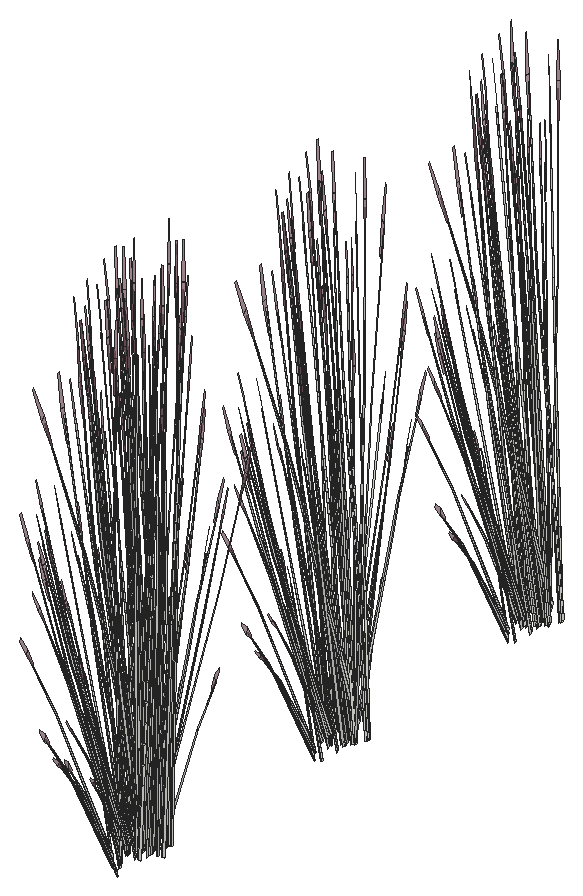
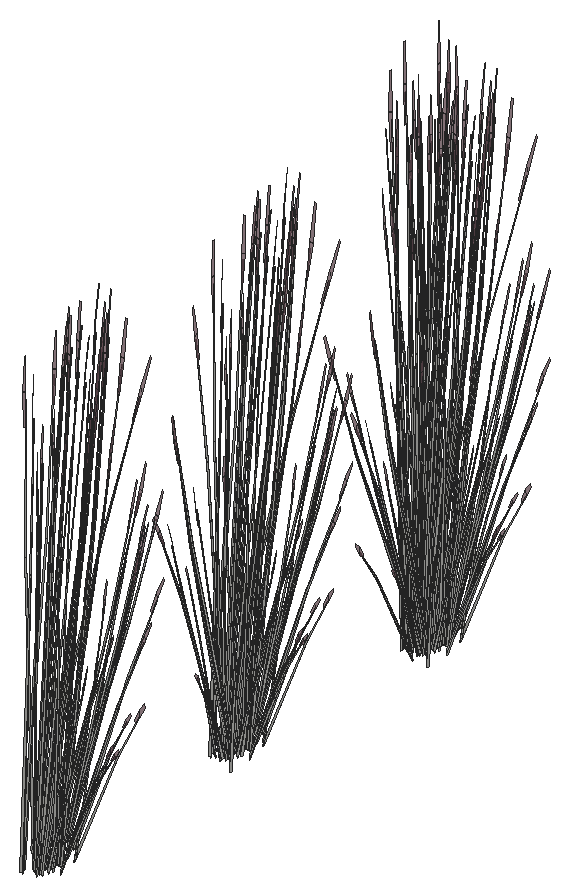
# SketchUp Ruby script. Lengths in inches.
U = 1.inch
M = Sketchup.active_model
def pt(a) = Geom::Point3d.new(a.map { |v| v * U })
def face(e, loops, mat)
  f = e.add_face(loops[0].map { |a| pt(a) })
  loops[1..].each { |l| e.add_face(l.map { |a| pt(a) }).erase! }
  f.material = f.back_material = mat if mat
  f
end
# faces: each face lists its corners as indices into pts; further lists are holes
def faces(e, pts, list, mat = nil) = list.each { |f| face(e, (f[0].is_a?(Array) ? f : [f]).map { |l| l.map { |i| pts[i] } }, mat) }
# xy, xz, yz: faces in a plane at the given z, y or x. An outline is a flat list of corners, or four numbers for a rectangle; further outlines are holes
def ring(l) = l.size == 4 ? [[l[0], l[1]], [l[2], l[1]], [l[2], l[3]], [l[0], l[3]]] : l.each_slice(2).to_a
def flat(e, list, mat, &to3) = list.each { |f| face(e, (f[0].is_a?(Array) ? f : [f]).map { |l| ring(l).map { |u, v| to3.(u, v) } }, mat) }
def xy(e, z, list, mat = nil) = flat(e, list, mat) { |x, y| [x, y, z] }
def xz(e, y, list, mat = nil) = flat(e, list, mat) { |x, z| [x, y, z] }
def yz(e, x, list, mat = nil) = flat(e, list, mat) { |y, z| [x, y, z] }
def lines(e, pts, list) = list.each { |a, b| e.add_line(pt(pts[a]), pt(pts[b])) }
# prism: a flat outline (further loops are holes) pulled along v
def prism(e, loops, v, mat = nil)
  f = face(e, loops, mat); d = Geom::Vector3d.new(v.map { |x| x * U })
  f.pushpull(f.normal.samedirection?(d) ? d.length : -d.length)
end
def box(e, o, s, mat = nil) = prism(e, [[o, [o[0] + s[0], o[1], o[2]], [o[0] + s[0], o[1] + s[1], o[2]], [o[0], o[1] + s[1], o[2]]]], [0, 0, s[2]], mat)
def at(x, y, z, deg = 0) = Geom::Transformation.translation(pt([x, y, z])) * Geom::Transformation.rotation(ORIGIN, Z_AXIS, deg.degrees)
def axes(o, x, y, z) = Geom::Transformation.new([*x, 0, *y, 0, *z, 0, *pt(o).to_a, 1])
def part(name) = M.definitions.add(name)
# library, detail: a bought-in or finely detailed component or shape, given as its bounding box
def library(name, o, s) = part(name).tap { |d| box(d.entities, o, s) }
def detail(e, o, s) = box(e.add_group.entities, o, s)
def put(e, d, t, mat = nil) = e.add_instance(d, t).tap { |i| i.material = mat if mat }
def group(e, t, mat = nil) = e.add_group.tap { |g| g.transformation = t; g.material = mat if mat }.entities
root = M.entities
M.materials.add("LightPink_Translucent").color = [144, 107, 117]
M.materials["LightPink_Translucent"].alpha = 0.75
c1 = part("blade")
p = [[2.15,0.21,22],[0,0.17,0],[0.09,0.45,0],[2.18,0.31,22],[2.29,0.31,22],[0.38,0.45,0],
  [2.48,0.24,33],[2.49,0.24,33],[2.48,0.22,33]]
faces(c1.entities,p,[[0,1,2,3],[4,5,2,3],[6,3,4,7],[8,0,3,6]])
c2 = part("seeds")
p = [[0.3,-0.1,1.38],[-0.01,-0.03,1.59],[-0.01,-0.03,0.03],[0.14,-0.07,-0.07],[0.29,-0.03,3],[0.15,0.01,3.11]]
faces(c2.entities,p,[[0,1,2,3],[1,0,4,5]],"LightPink_Translucent")
c3 = part("blade with seeds")
put(c3.entities,c1,at(0,0,0))
put(c3.entities,c2,axes([2.4,0.25,30.99],[1.5799,-0.05474,1.17369],[-0.12525,1.92788,0.29478],[-0.07173,-0.02425,1.56792]))
put(root,c3,axes([431.11,19.21,2.28],[-0.17959,-0.44867,-0.61099],[0.36969,-0.25004,0.07373],[-0.042,-0.21679,0.8643]))
put(root,c3,axes([429.9375,18.61,0.23],[-0.02279,0.18051,1.22981],[-0.33311,0.15111,-0.26449],[-0.07787,-0.23331,0.52581]))
put(root,c3,axes([430.8,18.21,-0.72],[-0.06312,0.01988,1.51654],[-0.34903,-0.22379,-0.23168],[0.00586,-0.18666,0.25832]))
put(root,c3,axes([431.14,18.83,1.89],[0.11344,-0.42434,-0.30456],[0.33096,0.12377,0.39319],[-0.03035,-0.17085,0.75234]))
put(root,c3,axes([430.97,19.12,2.03],[-0.3699,-0.13833,-0.43945],[0.12679,-0.47426,-0.34039],[-0.03392,-0.19095,0.84085]))
put(root,c3,axes([431.2,17.93,0.38],[0.04827,0.32177,0.9878],[-0.26778,-0.17821,0.72577],[0.02882,-0.16476,0.21757]))
put(root,c3,axes([429.82,18.32,0.38],[0.19628,0.19205,0.9878],[-0.28586,0.11545,0.72577],[-0.06116,-0.1476,0.21757]))
put(root,c3,axes([430.3,19.34,2.28],[-0.32086,-0.26671,-0.61099],[0.22803,-0.46737,0.07373],[-0.11625,-0.15925,0.8643]))
put(root,c3,axes([430.1875,18.98,1.89],[-0.05812,-0.44446,-0.30456],[0.33222,-0.11736,0.39319],[-0.08923,-0.12737,0.75234]))
put(root,c3,axes([429.67,18.9,-0.72],[-0.03645,0.07269,1.51654],[-0.36835,0.15672,-0.23168],[-0.08898,-0.14257,0.25832]))
put(root,c3,axes([430.28,20.9,-0.2],[-0.15453,-0.56584,-0.60058],[0.44514,-0.20379,-0.15763],[-0.01708,-0.19161,1.32568]))
put(root,c3,axes([430.15,19.35,2.03],[-0.37131,0.13117,-0.43945],[-0.06495,-0.49674,-0.34039],[-0.09973,-0.14235,0.84085]))
put(root,c3,axes([430.21,19.27,0.04],[-0.23526,-0.55293,0],[0.3936,-0.30836,-0.44382],[0.08964,-0.07023,1.40792]))
put(root,c3,axes([430.73,18.6,-0.17],[-0.26003,0.31656,-0.03348],[-0.23826,-0.3467,-0.15179],[-0.01677,-0.09824,0.50065]))
put(root,c3,axes([431.06,22.35,0.86],[0.32517,0.22251,1.30084],[-0.31856,0.47936,0.51441],[-0.14269,-0.28411,1.09053]))
put(root,c3,axes([429.36,20.82,-0.26],[0,-0.5518,-0.427],[0.42099,0,0],[0,-0.12568,1.35453]))
put(root,c3,axes([430.51,21.04,-0.1],[0.18257,-0.49721,-0.38476],[0.37935,0.23929,0.18517],[0,-0.11462,1.23533]))
put(root,c3,axes([429.42,19.77,1.89],[-0.2141,-0.34548,-0.30456],[0.24447,-0.32704,0.39319],[-0.12421,-0.04976,0.75234]))
put(root,c3,axes([429.55,20.83,-0.26],[0.26266,-0.34428,-0.26641],[0.26266,0.34428,0.26641],[0,-0.11089,1.19518]))
put(root,c3,axes([429.4375,19.18,-0.17],[-0.10855,0.45057,-0.03348],[-0.33409,-0.1386,-0.15179],[-0.05073,-0.0737,0.50065]))
put(root,c3,axes([430.47,21.45,0.29],[-0.42377,-0.26329,-0.25022],[0.20405,-0.55571,-0.43002],[-0.01332,-0.13644,1.37348]))
put(root,c3,axes([429.26,21.23,0.04],[-0.47052,0,0],[0,-0.61671,-0.44382],[0,-0.14046,1.40792]))
put(root,c3,axes([429.34,20.13,0.23],[0.07347,0.15363,1.22981],[-0.16929,0.41759,-0.26449],[-0.17383,-0.09981,0.52581]))
put(root,c3,axes([429.64,20,2.28],[-0.37615,-0.01329,-0.61099],[0.02526,-0.55946,0.07373],[-0.15935,-0.05904,0.8643]))
put(root,c3,axes([429.625,21.07,0],[-0.35001,0.46392,0.2645],[-0.35022,-0.45904,-0.31383],[-0.01222,-0.13174,1.41801]))
put(root,c3,axes([430.74,21.29,0.09],[0.42398,0.26744,0.20696],[-0.20405,0.55571,0.43002],[0,-0.1281,1.38067]))
put(root,c3,axes([430.57,22.04,0.1],[0.09973,-0.65385,-0.20149],[0.47288,0.11397,0.44093],[-0.08263,-0.0903,1.34539]))
put(root,c3,axes([429.52,20.11,2.03],[-0.27323,0.36552,-0.43945],[-0.23929,-0.38612,-0.34039],[-0.13882,-0.05561,0.84085]))
put(root,c3,axes([428.9,20.59,0.38],[0.24023,-0.03948,0.9878],[-0.15239,0.3479,0.72577],[-0.11872,-0.05219,0.21757]))
put(root,c3,axes([430.6,20.92,0.34],[-0.40861,0.03406,0.38476],[-0.03695,-0.56543,-0.18517],[0.07315,-0.05731,1.23533]))
put(root,c3,axes([429.55,21.33,0.13],[0,0.5518,0.427],[-0.42099,0,0],[0,-0.12568,1.35453]))
put(root,c3,axes([430.54,21.77,-0.1],[-0.22605,-0.46315,-0.38476],[0.34239,-0.32614,0.18517],[-0.07315,-0.05731,1.23533]))
put(root,c3,axes([430.59,21.12,0.03],[0.1636,0.61702,0.39349],[-0.46745,0.21456,0.15441],[0.00571,-0.11338,1.36617]))
put(root,c3,axes([430.5,21.61,0.34],[-0.18257,0.49721,0.38476],[-0.37935,-0.23929,-0.18517],[0,-0.11462,1.23533]))
put(root,c3,axes([431.17,21.17,-0.1],[0,-0.63847,0],[0.47052,0,0],[0,0,1.54332]))
put(root,c3,axes([430.34,21.95,-0.23],[-0.39143,-0.09047,-0.53624],[0.0826,-0.55804,-0.14074],[-0.11681,-0.06762,1.18365]))
put(root,c3,axes([430.95,20.77,0.03],[-0.312,0.50076,0.39349],[-0.37066,-0.44204,0.15441],[0.07522,-0.04998,1.36617]))
put(root,c3,axes([431.29,21.67,-0.02],[-0.35001,-0.47494,-0.05273],[0.35022,-0.47523,0],[-0.01222,-0.01659,1.50991]))
put(root,c3,axes([430.41,19.95,0.13],[-0.1087,0.54839,0.15172],[-0.39778,-0.15519,0.30174],[0.06871,-0.00267,1.3795]))
put(root,c3,axes([430.625,21.72,0.03],[0.4756,0.11626,0.39349],[-0.09679,0.6566,0.15441],[-0.0695,-0.0634,1.36617]))
put(root,c3,axes([429.08,21.16,-0.72],[0.00954,0.08696,1.51654],[-0.19238,0.45414,-0.23168],[-0.13665,-0.02289,0.25832]))
put(root,c3,axes([429.92,22.8,-0.26],[-0.08839,-0.48081,-0.26641],[0.35106,-0.13653,0.26641],[-0.07077,-0.05545,1.19518]))
put(root,c3,axes([430.37,22.77,0.13],[0.40434,-0.14646,0.15172],[0.09984,0.54504,0.30174],[-0.03606,-0.07941,1.3795]))
put(root,c3,axes([429.82,23.01,-0.26],[-0.35217,-0.2759,-0.427],[0.2105,-0.49473,0],[-0.08021,-0.06284,1.35453]))
put(root,c3,axes([429.04,20.97,1.89],[-0.31272,-0.15393,-0.30456],[0.09121,-0.44909,0.39319],[-0.1259,0.04118,0.75234]))
put(root,c3,axes([430.78,22.03,0.29],[-0.37992,0.36634,-0.25022],[-0.25264,-0.51764,-0.43002],[-0.09374,-0.05257,1.37348]))
put(root,c3,axes([431.61,19.98,0.13],[-0.40434,0.14646,0.15172],[-0.09984,-0.54504,0.30174],[0.03606,0.07941,1.3795]))
put(root,c3,axes([430.98,22.65,-0.1],[-0.12277,-0.47573,0],[0.35059,-0.1666,0],[0,0,1.32759]))
put(root,c3,axes([430.74,22.19,0.25],[-0.07259,0.49245,0.12452],[-0.35466,-0.08548,-0.35559],[-0.06454,-0.05057,1.09]))
put(root,c3,axes([431.57,22.8,0.13],[0.1087,-0.54839,0.15172],[0.39778,0.15519,0.30174],[-0.06871,0.00267,1.3795]))
put(root,c3,axes([429.99,20.89,0.875],[0.10696,-0.07982,1.52275],[0.03688,0.55733,0.11917],[-0.23167,0.07395,0.54424]))
put(root,c3,axes([432.2,21.4,0.13],[-0.29564,-0.40194,0.15172],[0.29793,-0.38985,0.30174],[-0.03265,0.08208,1.3795]))
put(root,c3,axes([430.89,22.86,-0.11],[-0.37935,-0.24773,0],[0.18257,-0.51475,0],[0,0,1.39928]))
put(root,c3,axes([431.21,22.2,0.12],[-0.36743,-0.44413,-0.21665],[0.30918,-0.49872,0.47412],[-0.09894,0.05195,1.44665]))
put(root,c3,axes([430.24,23.05,0.13],[0.35217,0.2759,0.427],[-0.2105,0.49473,0],[-0.08021,-0.06284,1.35453]))
put(root,c3,axes([431.41,21.43,-0.03],[0,0.63816,-0.04848],[-0.47052,0,0],[0,0.02005,1.54256]))
put(root,c3,axes([429.25,21.19,2.03],[-0.10194,0.50193,-0.43945],[-0.34951,-0.17204,-0.34039],[-0.14072,0.04602,0.84085]))
put(root,c3,axes([430.04,23.34,0.04],[-0.23526,0.55293,0],[-0.3936,-0.30836,-0.44382],[-0.08964,-0.07023,1.40792]))
put(root,c3,axes([431.38,21.83,0.34],[0.40861,-0.03406,0.38476],[0.03695,0.56543,-0.18517],[-0.07315,0.05731,1.23533]))
put(root,c3,axes([431.02,22.11,-0.1],[-0.40861,0.03406,-0.38476],[-0.03695,-0.56543,0.18517],[-0.07315,0.05731,1.23533]))
put(root,c3,axes([431.47,23.42,-0.11],[-0.23233,-0.55486,-0.04422],[0.3936,-0.30836,0.44382],[-0.09699,0.05283,1.40722]))
put(root,c3,axes([431.39,22.08,0.25],[0.278,0.33153,0.12452],[-0.23189,0.37404,-0.35559],[-0.06454,0.05057,1.09]))
put(root,c3,axes([431.6875,23.1,0.13],[0.35217,-0.2759,0.427],[0.2105,0.49473,0],[-0.08021,0.06284,1.35453]))
put(root,c3,axes([431.1875,22.66,-0.03],[0.1636,0.63392,-0.05171],[-0.46745,0.22213,0],[0.00571,0.02214,1.48069]))
put(root,c3,axes([431.37,23.35,-0.26],[-0.35106,-0.13653,-0.26641],[0.08839,-0.48081,0.26641],[-0.07077,0.05545,1.19518]))
put(root,c3,axes([428.83,22.37,0.23],[0.13077,0.0453,1.22981],[0.08428,0.46268,-0.26449],[-0.17763,0.08661,0.52581]))
put(root,c3,axes([432.54,21.83,-0.11],[-0.47029,-0.00441,-0.0428],[0,-0.61671,0.42951],[-0.01478,0.14039,1.36183]))
put(root,c3,axes([428.5625,23.34,0.38],[0.15682,-0.25009,0.9878],[0.06188,0.39591,0.72577],[-0.11333,0.07089,0.21757]))
put(root,c3,axes([431.31,21.95,0.29],[0.04385,0.62963,-0.25022],[-0.45669,0.03807,-0.43002],[-0.08042,0.08387,1.37348]))
put(root,c3,axes([431.47,21.71,-0.1],[-0.18257,0.49721,-0.38476],[-0.37935,-0.23929,0.18517],[0,0.11462,1.23533]))
put(root,c3,axes([429.15,22.26,1.89],[-0.32754,0.07886,-0.30456],[-0.08649,-0.45081,0.39319],[-0.09386,0.12109,0.75234]))
put(root,c3,axes([431.03,22.43,-0.23],[-0.25345,0.41475,-0.53624],[-0.31485,-0.37608,-0.14074],[-0.10156,0.10346,1.18365]))
put(root,c3,axes([431.48,23.13,0],[0.47108,0.17935,0.2645],[-0.11785,0.64108,-0.31383],[-0.07797,0.08023,1.41801]))
put(root,c3,axes([431.45,23.57,-0.26],[-0.35217,0.2759,-0.427],[-0.2105,-0.49473,0],[-0.08021,0.06284,1.35453]))
put(root,c3,axes([429.42,22.3125,2.03],[0.09666,0.50384,-0.43945],[-0.36608,0.08814,-0.34039],[-0.10491,0.13533,0.84085]))
put(root,c3,axes([431.77,23.48,0.04],[0.23526,0.55293,0],[-0.3936,0.30836,-0.44382],[-0.08964,0.07023,1.40792]))
put(root,c3,axes([431.57,21.29,0.44],[-0.01028,-0.51954,1.21494],[0.46521,0.13467,0.51441],[-0.11003,0.28429,1.14681]))
put(root,c3,axes([428.97,23.6,-0.72],[0.05047,0.05513,1.51654],[0.08558,0.51079,-0.23168],[-0.11187,0.10892,0.25832]))
put(root,c3,axes([429.73,23.3,1.89],[-0.2546,0.29052,-0.30456],[-0.24101,-0.33173,0.39319],[-0.03667,0.16855,0.75234]))
put(root,c3,axes([429.89,24.43,0.38],[-0.00974,-0.3281,0.9878],[0.24334,0.23402,0.72577],[-0.04786,0.15639,0.21757]))
put(root,c3,axes([430.53,23.65,-0.72],[0.0609,-0.03003,1.51654],[0.36632,0.16527,-0.23168],[0.01071,0.18627,0.25832]))
put(root,c3,axes([429.98,23.17,2.3],[0.26937,0.37076,-0.48779],[-0.28456,0.3247,-0.37783],[-0.04099,0.18838,0.93334]))
put(root,c3,axes([429.69,23.72,0.43],[0.34184,-0.09771,0.05596],[0.07859,0.39367,-0.74222],[-0.02167,0.19928,0.6653]))
put(root,c3,axes([430.61,23.82,1.89],[-0.11344,0.42434,-0.30456],[-0.33096,-0.12377,0.39319],[0.03035,0.17085,0.75234]))
put(root,c3,axes([429.9,23,2.59],[-0.00979,0.51041,-0.6782],[-0.4123,-0.03428,0.08184],[-0.04351,0.21623,0.95938]))
put(root,c3,axes([430.65,23.4375,2.28],[0.17959,0.44867,-0.61099],[-0.36969,0.25004,0.07373],[0.042,0.21679,0.8643]))
put(root,c3,axes([429.61,24.14,0.23],[0.11874,-0.08705,1.22981],[0.29317,0.26247,-0.26449],[-0.08726,0.22711,0.52581]))
put(root,c3,axes([429.76,23.72,0.89],[0.00827,-0.28486,1.32737],[0.37184,0.15046,0.18343],[-0.03222,0.30359,0.62678]))
put(root,c3,axes([432.74,42.25,2.28],[-0.17959,-0.44867,-0.61099],[0.36969,-0.25004,0.07373],[-0.042,-0.21679,0.8643]))
put(root,c3,axes([431.57,41.65,0.23],[-0.02279,0.18051,1.22981],[-0.33311,0.15111,-0.26449],[-0.07787,-0.23331,0.52581]))
put(root,c3,axes([432.6,42.16,2.03],[-0.3699,-0.13833,-0.43945],[0.12679,-0.47426,-0.34039],[-0.03392,-0.19095,0.84085]))
put(root,c3,axes([431.45,41.36,0.38],[0.19628,0.19205,0.9878],[-0.28586,0.11545,0.72577],[-0.06116,-0.1476,0.21757]))
put(root,c3,axes([431.93,42.38,2.28],[-0.32086,-0.26671,-0.61099],[0.22803,-0.46737,0.07373],[-0.11625,-0.15925,0.8643]))
put(root,c3,axes([431.82,42.03,1.89],[-0.05812,-0.44446,-0.30456],[0.33222,-0.11736,0.39319],[-0.08923,-0.12737,0.75234]))
put(root,c3,axes([431.3,41.94,-0.72],[-0.03645,0.07269,1.51654],[-0.36835,0.15672,-0.23168],[-0.08898,-0.14257,0.25832]))
put(root,c3,axes([431.9,43.9375,-0.2],[-0.15453,-0.56584,-0.60058],[0.44514,-0.20379,-0.15763],[-0.01708,-0.19161,1.32568]))
put(root,c3,axes([431.78,42.39,2.03],[-0.37131,0.13117,-0.43945],[-0.06495,-0.49674,-0.34039],[-0.09973,-0.14235,0.84085]))
put(root,c3,axes([432.36,41.64,-0.17],[-0.26003,0.31656,-0.03348],[-0.23826,-0.3467,-0.15179],[-0.01677,-0.09824,0.50065]))
put(root,c3,axes([432.69,45.4,0.86],[0.32517,0.22251,1.30084],[-0.31856,0.47936,0.51441],[-0.14269,-0.28411,1.09053]))
put(root,c3,axes([430.99,43.86,-0.26],[0,-0.5518,-0.427],[0.42099,0,0],[0,-0.12568,1.35453]))
put(root,c3,axes([431.05,42.81,1.89],[-0.2141,-0.34548,-0.30456],[0.24447,-0.32704,0.39319],[-0.12421,-0.04976,0.75234]))
put(root,c3,axes([431.17,43.87,-0.26],[0.26266,-0.34428,-0.26641],[0.26266,0.34428,0.26641],[0,-0.11089,1.19518]))
put(root,c3,axes([431.07,42.22,-0.17],[-0.10855,0.45057,-0.03348],[-0.33409,-0.1386,-0.15179],[-0.05073,-0.0737,0.50065]))
put(root,c3,axes([432.09,44.5,0.29],[-0.42377,-0.26329,-0.25022],[0.20405,-0.55571,-0.43002],[-0.01332,-0.13644,1.37348]))
put(root,c3,axes([430.89,44.28,0.04],[-0.47052,0,0],[0,-0.61671,-0.44382],[0,-0.14046,1.40792]))
put(root,c3,axes([430.97,43.17,0.23],[0.07347,0.15363,1.22981],[-0.16929,0.41759,-0.26449],[-0.17383,-0.09981,0.52581]))
put(root,c3,axes([431.27,43.04,2.28],[-0.37615,-0.01329,-0.61099],[0.02526,-0.55946,0.07373],[-0.15935,-0.05904,0.8643]))
put(root,c3,axes([431.25,44.11,0],[-0.35001,0.46392,0.2645],[-0.35022,-0.45904,-0.31383],[-0.01222,-0.13174,1.41801]))
put(root,c3,axes([432.2,45.08,0.1],[0.09973,-0.65385,-0.20149],[0.47288,0.11397,0.44093],[-0.08263,-0.0903,1.34539]))
put(root,c3,axes([431.15,43.15,2.03],[-0.27323,0.36552,-0.43945],[-0.23929,-0.38612,-0.34039],[-0.13882,-0.05561,0.84085]))
put(root,c3,axes([430.53,43.64,0.38],[0.24023,-0.03948,0.9878],[-0.15239,0.3479,0.72577],[-0.11872,-0.05219,0.21757]))
put(root,c3,axes([431.17,44.37,0.13],[0,0.5518,0.427],[-0.42099,0,0],[0,-0.12568,1.35453]))
put(root,c3,axes([432.17,44.82,-0.1],[-0.22605,-0.46315,-0.38476],[0.34239,-0.32614,0.18517],[-0.07315,-0.05731,1.23533]))
put(root,c3,axes([432.13,44.65,0.34],[-0.18257,0.49721,0.38476],[-0.37935,-0.23929,-0.18517],[0,-0.11462,1.23533]))
put(root,c3,axes([431.97,44.99,-0.23],[-0.39143,-0.09047,-0.53624],[0.0826,-0.55804,-0.14074],[-0.11681,-0.06762,1.18365]))
put(root,c3,axes([432.26,44.77,0.03],[0.4756,0.11626,0.39349],[-0.09679,0.6566,0.15441],[-0.0695,-0.0634,1.36617]))
put(root,c3,axes([430.71,44.2,-0.72],[0.00954,0.08696,1.51654],[-0.19238,0.45414,-0.23168],[-0.13665,-0.02289,0.25832]))
put(root,c3,axes([431.55,45.84,-0.26],[-0.08839,-0.48081,-0.26641],[0.35106,-0.13653,0.26641],[-0.07077,-0.05545,1.19518]))
put(root,c3,axes([431.45,46.05,-0.26],[-0.35217,-0.2759,-0.427],[0.2105,-0.49473,0],[-0.08021,-0.06284,1.35453]))
put(root,c3,axes([430.67,44.01,1.89],[-0.31272,-0.15393,-0.30456],[0.09121,-0.44909,0.39319],[-0.1259,0.04118,0.75234]))
put(root,c3,axes([432.41,45.08,0.29],[-0.37992,0.36634,-0.25022],[-0.25264,-0.51764,-0.43002],[-0.09374,-0.05257,1.37348]))
put(root,c3,axes([432.375,45.24,0.25],[-0.07259,0.49245,0.12452],[-0.35466,-0.08548,-0.35559],[-0.06454,-0.05057,1.09]))
put(root,c3,axes([431.62,43.93,0.875],[0.10696,-0.07982,1.52275],[0.03688,0.55733,0.11917],[-0.23167,0.07395,0.54424]))
put(root,c3,axes([432.84,45.24,0.12],[-0.36743,-0.44413,-0.21665],[0.30918,-0.49872,0.47412],[-0.09894,0.05195,1.44665]))
put(root,c3,axes([431.87,46.09,0.13],[0.35217,0.2759,0.427],[-0.2105,0.49473,0],[-0.08021,-0.06284,1.35453]))
put(root,c3,axes([430.88,44.24,2.03],[-0.10194,0.50193,-0.43945],[-0.34951,-0.17204,-0.34039],[-0.14072,0.04602,0.84085]))
put(root,c3,axes([431.67,46.38,0.04],[-0.23526,0.55293,0],[-0.3936,-0.30836,-0.44382],[-0.08964,-0.07023,1.40792]))
put(root,c3,axes([432.65,45.15,-0.1],[-0.40861,0.03406,-0.38476],[-0.03695,-0.56543,0.18517],[-0.07315,0.05731,1.23533]))
put(root,c3,axes([433.1,46.46,-0.11],[-0.23233,-0.55486,-0.04422],[0.3936,-0.30836,0.44382],[-0.09699,0.05283,1.40722]))
put(root,c3,axes([433,46.39,-0.26],[-0.35106,-0.13653,-0.26641],[0.08839,-0.48081,0.26641],[-0.07077,0.05545,1.19518]))
put(root,c3,axes([430.46,45.41,0.23],[0.13077,0.0453,1.22981],[0.08428,0.46268,-0.26449],[-0.17763,0.08661,0.52581]))
put(root,c3,axes([430.19,46.38,0.38],[0.15682,-0.25009,0.9878],[0.06188,0.39591,0.72577],[-0.11333,0.07089,0.21757]))
put(root,c3,axes([432.9375,44.99,0.29],[0.04385,0.62963,-0.25022],[-0.45669,0.03807,-0.43002],[-0.08042,0.08387,1.37348]))
put(root,c3,axes([430.78,45.3,1.89],[-0.32754,0.07886,-0.30456],[-0.08649,-0.45081,0.39319],[-0.09386,0.12109,0.75234]))
put(root,c3,axes([432.66,45.48,-0.23],[-0.25345,0.41475,-0.53624],[-0.31485,-0.37608,-0.14074],[-0.10156,0.10346,1.18365]))
put(root,c3,axes([433.08,46.61,-0.26],[-0.35217,0.2759,-0.427],[-0.2105,-0.49473,0],[-0.08021,0.06284,1.35453]))
put(root,c3,axes([431.05,45.35,2.03],[0.09666,0.50384,-0.43945],[-0.36608,0.08814,-0.34039],[-0.10491,0.13533,0.84085]))
put(root,c3,axes([433.2,44.33,0.44],[-0.01028,-0.51954,1.21494],[0.46521,0.13467,0.51441],[-0.11003,0.28429,1.14681]))
put(root,c3,axes([430.6,46.64,-0.72],[0.05047,0.05513,1.51654],[0.08558,0.51079,-0.23168],[-0.11187,0.10892,0.25832]))
put(root,c3,axes([431.36,46.35,1.89],[-0.2546,0.29052,-0.30456],[-0.24101,-0.33173,0.39319],[-0.03667,0.16855,0.75234]))
put(root,c3,axes([431.52,47.47,0.38],[-0.00974,-0.3281,0.9878],[0.24334,0.23402,0.72577],[-0.04786,0.15639,0.21757]))
put(root,c3,axes([431.61,46.21,2.3],[0.26937,0.37076,-0.48779],[-0.28456,0.3247,-0.37783],[-0.04099,0.18838,0.93334]))
put(root,c3,axes([431.32,46.76,0.43],[0.34184,-0.09771,0.05596],[0.07859,0.39367,-0.74222],[-0.02167,0.19928,0.6653]))
put(root,c3,axes([431.53,46.04,2.59],[-0.00979,0.51041,-0.6782],[-0.4123,-0.03428,0.08184],[-0.04351,0.21623,0.95938]))
put(root,c3,axes([431.24,47.18,0.23],[0.11874,-0.08705,1.22981],[0.29317,0.26247,-0.26449],[-0.08726,0.22711,0.52581]))
put(root,c3,axes([431.39,46.76,0.89],[0.00827,-0.28486,1.32737],[0.37184,0.15046,0.18343],[-0.03222,0.30359,0.62678]))
put(root,c3,axes([432.74,66.25,2.28],[-0.17959,-0.44867,-0.61099],[0.36969,-0.25004,0.07373],[-0.042,-0.21679,0.8643]))
put(root,c3,axes([431.57,65.65,0.23],[-0.02279,0.18051,1.22981],[-0.33311,0.15111,-0.26449],[-0.07787,-0.23331,0.52581]))
put(root,c3,axes([432.6,66.16,2.03],[-0.3699,-0.13833,-0.43945],[0.12679,-0.47426,-0.34039],[-0.03392,-0.19095,0.84085]))
put(root,c3,axes([431.45,65.36,0.38],[0.19628,0.19205,0.9878],[-0.28586,0.11545,0.72577],[-0.06116,-0.1476,0.21757]))
put(root,c3,axes([431.93,66.38,2.28],[-0.32086,-0.26671,-0.61099],[0.22803,-0.46737,0.07373],[-0.11625,-0.15925,0.8643]))
put(root,c3,axes([431.82,66.03,1.89],[-0.05812,-0.44446,-0.30456],[0.33222,-0.11736,0.39319],[-0.08923,-0.12737,0.75234]))
put(root,c3,axes([431.3,65.94,-0.72],[-0.03645,0.07269,1.51654],[-0.36835,0.15672,-0.23168],[-0.08898,-0.14257,0.25832]))
put(root,c3,axes([431.9,67.9375,-0.2],[-0.15453,-0.56584,-0.60058],[0.44514,-0.20379,-0.15763],[-0.01708,-0.19161,1.32568]))
put(root,c3,axes([431.78,66.39,2.03],[-0.37131,0.13117,-0.43945],[-0.06495,-0.49674,-0.34039],[-0.09973,-0.14235,0.84085]))
put(root,c3,axes([432.36,65.64,-0.17],[-0.26003,0.31656,-0.03348],[-0.23826,-0.3467,-0.15179],[-0.01677,-0.09824,0.50065]))
put(root,c3,axes([432.69,69.4,0.86],[0.32517,0.22251,1.30084],[-0.31856,0.47936,0.51441],[-0.14269,-0.28411,1.09053]))
put(root,c3,axes([430.99,67.86,-0.26],[0,-0.5518,-0.427],[0.42099,0,0],[0,-0.12568,1.35453]))
put(root,c3,axes([431.05,66.81,1.89],[-0.2141,-0.34548,-0.30456],[0.24447,-0.32704,0.39319],[-0.12421,-0.04976,0.75234]))
put(root,c3,axes([431.17,67.87,-0.26],[0.26266,-0.34428,-0.26641],[0.26266,0.34428,0.26641],[0,-0.11089,1.19518]))
put(root,c3,axes([431.07,66.22,-0.17],[-0.10855,0.45057,-0.03348],[-0.33409,-0.1386,-0.15179],[-0.05073,-0.0737,0.50065]))
put(root,c3,axes([432.09,68.5,0.29],[-0.42377,-0.26329,-0.25022],[0.20405,-0.55571,-0.43002],[-0.01332,-0.13644,1.37348]))
put(root,c3,axes([430.89,68.28,0.04],[-0.47052,0,0],[0,-0.61671,-0.44382],[0,-0.14046,1.40792]))
put(root,c3,axes([430.97,67.17,0.23],[0.07347,0.15363,1.22981],[-0.16929,0.41759,-0.26449],[-0.17383,-0.09981,0.52581]))
put(root,c3,axes([431.27,67.04,2.28],[-0.37615,-0.01329,-0.61099],[0.02526,-0.55946,0.07373],[-0.15935,-0.05904,0.8643]))
put(root,c3,axes([431.25,68.11,0],[-0.35001,0.46392,0.2645],[-0.35022,-0.45904,-0.31383],[-0.01222,-0.13174,1.41801]))
put(root,c3,axes([432.2,69.08,0.1],[0.09973,-0.65385,-0.20149],[0.47288,0.11397,0.44093],[-0.08263,-0.0903,1.34539]))
put(root,c3,axes([431.15,67.15,2.03],[-0.27323,0.36552,-0.43945],[-0.23929,-0.38612,-0.34039],[-0.13882,-0.05561,0.84085]))
put(root,c3,axes([430.53,67.64,0.38],[0.24023,-0.03948,0.9878],[-0.15239,0.3479,0.72577],[-0.11872,-0.05219,0.21757]))
put(root,c3,axes([431.17,68.37,0.13],[0,0.5518,0.427],[-0.42099,0,0],[0,-0.12568,1.35453]))
put(root,c3,axes([432.17,68.82,-0.1],[-0.22605,-0.46315,-0.38476],[0.34239,-0.32614,0.18517],[-0.07315,-0.05731,1.23533]))
put(root,c3,axes([432.13,68.65,0.34],[-0.18257,0.49721,0.38476],[-0.37935,-0.23929,-0.18517],[0,-0.11462,1.23533]))
put(root,c3,axes([431.97,68.99,-0.23],[-0.39143,-0.09047,-0.53624],[0.0826,-0.55804,-0.14074],[-0.11681,-0.06762,1.18365]))
put(root,c3,axes([432.26,68.77,0.03],[0.4756,0.11626,0.39349],[-0.09679,0.6566,0.15441],[-0.0695,-0.0634,1.36617]))
put(root,c3,axes([430.71,68.2,-0.72],[0.00954,0.08696,1.51654],[-0.19238,0.45414,-0.23168],[-0.13665,-0.02289,0.25832]))
put(root,c3,axes([431.55,69.84,-0.26],[-0.08839,-0.48081,-0.26641],[0.35106,-0.13653,0.26641],[-0.07077,-0.05545,1.19518]))
put(root,c3,axes([431.45,70.05,-0.26],[-0.35217,-0.2759,-0.427],[0.2105,-0.49473,0],[-0.08021,-0.06284,1.35453]))
put(root,c3,axes([430.67,68.01,1.89],[-0.31272,-0.15393,-0.30456],[0.09121,-0.44909,0.39319],[-0.1259,0.04118,0.75234]))
put(root,c3,axes([432.41,69.08,0.29],[-0.37992,0.36634,-0.25022],[-0.25264,-0.51764,-0.43002],[-0.09374,-0.05257,1.37348]))
put(root,c3,axes([432.375,69.24,0.25],[-0.07259,0.49245,0.12452],[-0.35466,-0.08548,-0.35559],[-0.06454,-0.05057,1.09]))
put(root,c3,axes([431.62,67.93,0.875],[0.10696,-0.07982,1.52275],[0.03688,0.55733,0.11917],[-0.23167,0.07395,0.54424]))
put(root,c3,axes([432.84,69.24,0.12],[-0.36743,-0.44413,-0.21665],[0.30918,-0.49872,0.47412],[-0.09894,0.05195,1.44665]))
put(root,c3,axes([431.87,70.09,0.13],[0.35217,0.2759,0.427],[-0.2105,0.49473,0],[-0.08021,-0.06284,1.35453]))
put(root,c3,axes([430.88,68.24,2.03],[-0.10194,0.50193,-0.43945],[-0.34951,-0.17204,-0.34039],[-0.14072,0.04602,0.84085]))
put(root,c3,axes([431.67,70.38,0.04],[-0.23526,0.55293,0],[-0.3936,-0.30836,-0.44382],[-0.08964,-0.07023,1.40792]))
put(root,c3,axes([432.65,69.15,-0.1],[-0.40861,0.03406,-0.38476],[-0.03695,-0.56543,0.18517],[-0.07315,0.05731,1.23533]))
put(root,c3,axes([433.1,70.46,-0.11],[-0.23233,-0.55486,-0.04422],[0.3936,-0.30836,0.44382],[-0.09699,0.05283,1.40722]))
put(root,c3,axes([433,70.39,-0.26],[-0.35106,-0.13653,-0.26641],[0.08839,-0.48081,0.26641],[-0.07077,0.05545,1.19518]))
put(root,c3,axes([430.46,69.41,0.23],[0.13077,0.0453,1.22981],[0.08428,0.46268,-0.26449],[-0.17763,0.08661,0.52581]))
put(root,c3,axes([430.19,70.38,0.38],[0.15682,-0.25009,0.9878],[0.06188,0.39591,0.72577],[-0.11333,0.07089,0.21757]))
put(root,c3,axes([432.9375,68.99,0.29],[0.04385,0.62963,-0.25022],[-0.45669,0.03807,-0.43002],[-0.08042,0.08387,1.37348]))
put(root,c3,axes([430.78,69.3,1.89],[-0.32754,0.07886,-0.30456],[-0.08649,-0.45081,0.39319],[-0.09386,0.12109,0.75234]))
put(root,c3,axes([432.66,69.48,-0.23],[-0.25345,0.41475,-0.53624],[-0.31485,-0.37608,-0.14074],[-0.10156,0.10346,1.18365]))
put(root,c3,axes([433.08,70.61,-0.26],[-0.35217,0.2759,-0.427],[-0.2105,-0.49473,0],[-0.08021,0.06284,1.35453]))
